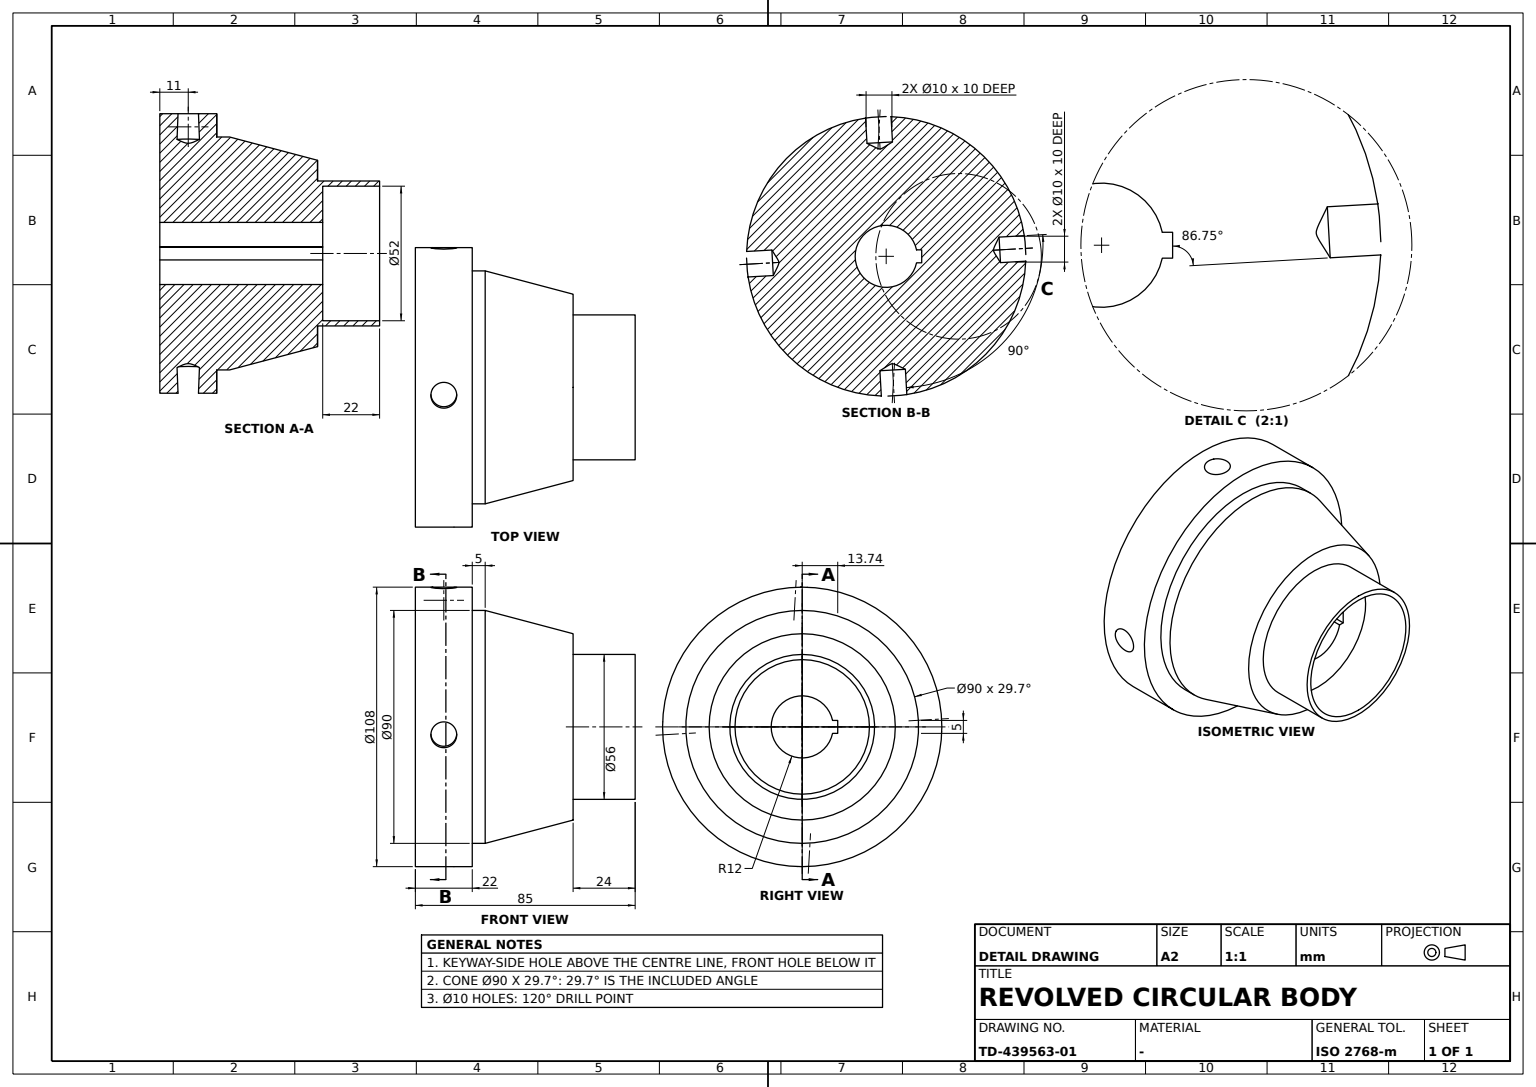
ISO-10303-21;
HEADER;
FILE_DESCRIPTION((''),'2;1');
FILE_NAME('','',(''),(''),'','','');
FILE_SCHEMA(('AUTOMOTIVE_DESIGN'));
ENDSEC;
DATA;
#1=APPLICATION_CONTEXT('');
#2=PRODUCT_CONTEXT('',#1,'mechanical');
#3=PRODUCT('','','',(#2));
#4=PRODUCT_DEFINITION_FORMATION('','',#3);
#5=PRODUCT_DEFINITION_CONTEXT('',#1,'design');
#6=PRODUCT_DEFINITION('','',#4,#5);
#7=PRODUCT_DEFINITION_SHAPE('','',#6);
#8=(LENGTH_UNIT()NAMED_UNIT(*)SI_UNIT(.MILLI.,.METRE.));
#9=(NAMED_UNIT(*)PLANE_ANGLE_UNIT()SI_UNIT($,.RADIAN.));
#10=(NAMED_UNIT(*)SI_UNIT($,.STERADIAN.)SOLID_ANGLE_UNIT());
#11=UNCERTAINTY_MEASURE_WITH_UNIT(LENGTH_MEASURE(0.005),#8,'distance_accuracy_value','');
#12=(GEOMETRIC_REPRESENTATION_CONTEXT(3)GLOBAL_UNCERTAINTY_ASSIGNED_CONTEXT((#11))GLOBAL_UNIT_ASSIGNED_CONTEXT((#8,#9,#10))REPRESENTATION_CONTEXT('',''));
#13=CARTESIAN_POINT('',(-78.387913,-0.666342,53.995889));
#14=VERTEX_POINT('',#13);
#15=CARTESIAN_POINT('',(-79.315768,-4.629244,53.854393));
#16=CARTESIAN_POINT('',(-78.86274,-0.407001,54.04207));
#17=CARTESIAN_POINT('',(-75.560747,2.259197,53.952659));
#18=CARTESIAN_POINT('',(-71.347706,1.80512,53.979216));
#19=CARTESIAN_POINT('',(-68.68427,-1.499404,54.032185));
#20=CARTESIAN_POINT('',(-69.13719,-5.715656,53.740509));
#21=CARTESIAN_POINT('',(-72.439195,-8.354711,53.349717));
#22=CARTESIAN_POINT('',(-76.652299,-7.906564,53.427525));
#23=B_SPLINE_CURVE_WITH_KNOTS('',3,(#15,#16,#17,#18,#19,#20,#21,#22,#15,#16,#17),.UNSPECIFIED.,.T.,.F.,(1,1,1,1,1,1,1,1,1,1,1,1,1,1,1),(-0.01172778,-0.00781852,-0.00390926,0.,0.00390926,0.00781852,0.01172778,0.01563704,0.0195463,0.02345556,0.02736482,0.03127408,0.035183339,0.039092599,0.043001859),.UNSPECIFIED.);
#24=EDGE_CURVE('',#14,#14,#23,.T.);
#25=ORIENTED_EDGE('',*,*,#24,.F.);
#26=EDGE_LOOP('',(#25));
#27=FACE_BOUND('',#26,.T.);
#28=CARTESIAN_POINT('',(-74.,-7.487428,43.6456));
#29=VERTEX_POINT('',#28);
#30=CARTESIAN_POINT('',(-74.,-2.495477,43.929177));
#31=DIRECTION('',(0.,-0.056715376,0.998390388));
#32=DIRECTION('',(0.,-0.998390388,-0.056715376));
#33=AXIS2_PLACEMENT_3D('',#30,#31,#32);
#34=CIRCLE('',#33,5.);
#35=EDGE_CURVE('',#29,#29,#34,.F.);
#36=ORIENTED_EDGE('',*,*,#35,.T.);
#37=EDGE_LOOP('',(#36));
#38=FACE_BOUND('',#37,.T.);
#39=CARTESIAN_POINT('',(-74.,-3.056959,53.813242));
#40=DIRECTION('',(0.,0.056715376,-0.998390388));
#41=DIRECTION('',(1.,0.,0.));
#42=AXIS2_PLACEMENT_3D('',#39,#40,#41);
#43=CYLINDRICAL_SURFACE('',#42,5.);
#44=ADVANCED_FACE('',(#27,#38),#43,.F.);
#45=ORIENTED_EDGE('',*,*,#35,.F.);
#46=EDGE_LOOP('',(#45));
#47=FACE_BOUND('',#46,.T.);
#48=CARTESIAN_POINT('',(-74.,-2.331753,41.047072));
#49=VERTEX_POINT('',#48);
#50=VERTEX_LOOP('',#49);
#51=FACE_BOUND('',#50,.T.);
#52=AXIS2_PLACEMENT_3D('',#48,#31,#41);
#53=CONICAL_SURFACE('',#52,0.,1.047197551);
#54=ADVANCED_FACE('',(#47,#51),#53,.F.);
#55=CARTESIAN_POINT('',(-74.,43.6456,7.487428));
#56=VERTEX_POINT('',#55);
#57=CARTESIAN_POINT('',(-74.,43.929177,2.495477));
#58=DIRECTION('',(0.,0.998390388,0.056715376));
#59=AXIS2_PLACEMENT_3D('',#57,#58,#31);
#60=CIRCLE('',#59,5.);
#61=EDGE_CURVE('',#56,#56,#60,.F.);
#62=ORIENTED_EDGE('',*,*,#61,.F.);
#63=EDGE_LOOP('',(#62));
#64=FACE_BOUND('',#63,.T.);
#65=CARTESIAN_POINT('',(-74.,41.047072,2.331753));
#66=VERTEX_POINT('',#65);
#67=VERTEX_LOOP('',#66);
#68=FACE_BOUND('',#67,.T.);
#69=AXIS2_PLACEMENT_3D('',#65,#58,#41);
#70=CONICAL_SURFACE('',#69,0.,1.047197551);
#71=ADVANCED_FACE('',(#64,#68),#70,.F.);
#72=CARTESIAN_POINT('',(-24.,0.,28.));
#73=VERTEX_POINT('',#72);
#74=CARTESIAN_POINT('',(-24.,0.,0.));
#75=DIRECTION('',(-1.,0.,0.));
#76=DIRECTION('',(0.,0.,1.));
#77=AXIS2_PLACEMENT_3D('',#74,#75,#76);
#78=CIRCLE('',#77,28.);
#79=EDGE_CURVE('',#73,#73,#78,.T.);
#80=ORIENTED_EDGE('',*,*,#79,.F.);
#81=EDGE_LOOP('',(#80));
#82=FACE_BOUND('',#81,.T.);
#83=CARTESIAN_POINT('',(0.,0.,28.));
#84=VERTEX_POINT('',#83);
#85=CARTESIAN_POINT('',(0.,0.,0.));
#86=AXIS2_PLACEMENT_3D('',#85,#75,#76);
#87=CIRCLE('',#86,28.);
#88=EDGE_CURVE('',#84,#84,#87,.T.);
#89=ORIENTED_EDGE('',*,*,#88,.T.);
#90=EDGE_LOOP('',(#89));
#91=FACE_BOUND('',#90,.T.);
#92=CARTESIAN_POINT('',(-42.5,0.,0.));
#93=DIRECTION('',(0.,1.,0.));
#94=AXIS2_PLACEMENT_3D('',#92,#75,#93);
#95=CYLINDRICAL_SURFACE('',#94,28.);
#96=ADVANCED_FACE('',(#82,#91),#95,.T.);
#97=CARTESIAN_POINT('',(-24.,0.,36.));
#98=VERTEX_POINT('',#97);
#99=CIRCLE('',#77,36.);
#100=EDGE_CURVE('',#98,#98,#99,.T.);
#101=ORIENTED_EDGE('',*,*,#100,.F.);
#102=EDGE_LOOP('',(#101));
#103=FACE_BOUND('',#102,.T.);
#104=ORIENTED_EDGE('',*,*,#79,.T.);
#105=EDGE_LOOP('',(#104));
#106=FACE_BOUND('',#105,.T.);
#107=AXIS2_PLACEMENT_3D('',#97,#75,#93);
#108=PLANE('',#107);
#109=ADVANCED_FACE('',(#103,#106),#108,.F.);
#110=ORIENTED_EDGE('',*,*,#100,.T.);
#111=EDGE_LOOP('',(#110));
#112=FACE_BOUND('',#111,.T.);
#113=CARTESIAN_POINT('',(-58.,0.,45.));
#114=VERTEX_POINT('',#113);
#115=CARTESIAN_POINT('',(-58.,0.,0.));
#116=AXIS2_PLACEMENT_3D('',#115,#75,#76);
#117=CIRCLE('',#116,45.);
#118=EDGE_CURVE('',#114,#114,#117,.T.);
#119=ORIENTED_EDGE('',*,*,#118,.F.);
#120=EDGE_LOOP('',(#119));
#121=FACE_BOUND('',#120,.T.);
#122=AXIS2_PLACEMENT_3D('',#74,#75,#93);
#123=CONICAL_SURFACE('',#122,36.,0.258770892);
#124=ADVANCED_FACE('',(#112,#121),#123,.T.);
#125=CARTESIAN_POINT('',(-74.,2.331753,-41.047072));
#126=VERTEX_POINT('',#125);
#127=VERTEX_LOOP('',#126);
#128=FACE_BOUND('',#127,.T.);
#129=CARTESIAN_POINT('',(-74.,7.487428,-43.6456));
#130=VERTEX_POINT('',#129);
#131=CARTESIAN_POINT('',(-74.,2.495477,-43.929177));
#132=AXIS2_PLACEMENT_3D('',#131,#40,#58);
#133=CIRCLE('',#132,5.);
#134=EDGE_CURVE('',#130,#130,#133,.F.);
#135=ORIENTED_EDGE('',*,*,#134,.F.);
#136=EDGE_LOOP('',(#135));
#137=FACE_BOUND('',#136,.T.);
#138=AXIS2_PLACEMENT_3D('',#125,#40,#41);
#139=CONICAL_SURFACE('',#138,0.,1.047197551);
#140=ADVANCED_FACE('',(#128,#137),#139,.F.);
#141=CARTESIAN_POINT('',(-78.387913,53.995889,0.666342));
#142=VERTEX_POINT('',#141);
#143=CARTESIAN_POINT('',(-79.315768,53.854393,4.629244));
#144=CARTESIAN_POINT('',(-78.86274,54.04207,0.407001));
#145=CARTESIAN_POINT('',(-75.560747,53.952659,-2.259197));
#146=CARTESIAN_POINT('',(-71.347706,53.979216,-1.80512));
#147=CARTESIAN_POINT('',(-68.68427,54.032185,1.499404));
#148=CARTESIAN_POINT('',(-69.13719,53.740509,5.715656));
#149=CARTESIAN_POINT('',(-72.439195,53.349717,8.354711));
#150=CARTESIAN_POINT('',(-76.652299,53.427525,7.906564));
#151=B_SPLINE_CURVE_WITH_KNOTS('',3,(#143,#144,#145,#146,#147,#148,#149,#150,#143,#144,#145),.UNSPECIFIED.,.T.,.F.,(1,1,1,1,1,1,1,1,1,1,1,1,1,1,1),(-0.01172778,-0.00781852,-0.00390926,0.,0.00390926,0.00781852,0.01172778,0.01563704,0.0195463,0.02345556,0.02736482,0.03127408,0.035183339,0.039092599,0.043001859),.UNSPECIFIED.);
#152=EDGE_CURVE('',#142,#142,#151,.T.);
#153=ORIENTED_EDGE('',*,*,#152,.F.);
#154=EDGE_LOOP('',(#153));
#155=FACE_BOUND('',#154,.T.);
#156=ORIENTED_EDGE('',*,*,#61,.T.);
#157=EDGE_LOOP('',(#156));
#158=FACE_BOUND('',#157,.T.);
#159=CARTESIAN_POINT('',(-74.,53.813242,3.056959));
#160=AXIS2_PLACEMENT_3D('',#159,#32,#41);
#161=CYLINDRICAL_SURFACE('',#160,5.);
#162=ADVANCED_FACE('',(#155,#158),#161,.F.);
#163=CARTESIAN_POINT('',(-78.387913,0.666342,-53.995889));
#164=VERTEX_POINT('',#163);
#165=CARTESIAN_POINT('',(-79.315768,4.629244,-53.854393));
#166=CARTESIAN_POINT('',(-78.86274,0.407001,-54.04207));
#167=CARTESIAN_POINT('',(-75.560747,-2.259197,-53.952659));
#168=CARTESIAN_POINT('',(-71.347706,-1.80512,-53.979216));
#169=CARTESIAN_POINT('',(-68.68427,1.499404,-54.032185));
#170=CARTESIAN_POINT('',(-69.13719,5.715656,-53.740509));
#171=CARTESIAN_POINT('',(-72.439195,8.354711,-53.349717));
#172=CARTESIAN_POINT('',(-76.652299,7.906564,-53.427525));
#173=B_SPLINE_CURVE_WITH_KNOTS('',3,(#165,#166,#167,#168,#169,#170,#171,#172,#165,#166,#167),.UNSPECIFIED.,.T.,.F.,(1,1,1,1,1,1,1,1,1,1,1,1,1,1,1),(-0.01172778,-0.00781852,-0.00390926,0.,0.00390926,0.00781852,0.01172778,0.01563704,0.0195463,0.02345556,0.02736482,0.03127408,0.035183339,0.039092599,0.043001859),.UNSPECIFIED.);
#174=EDGE_CURVE('',#164,#164,#173,.T.);
#175=ORIENTED_EDGE('',*,*,#174,.T.);
#176=EDGE_LOOP('',(#175));
#177=FACE_BOUND('',#176,.T.);
#178=CARTESIAN_POINT('',(-63.,0.,54.));
#179=VERTEX_POINT('',#178);
#180=CARTESIAN_POINT('',(-63.,0.,0.));
#181=AXIS2_PLACEMENT_3D('',#180,#75,#76);
#182=CIRCLE('',#181,54.);
#183=EDGE_CURVE('',#179,#179,#182,.T.);
#184=ORIENTED_EDGE('',*,*,#183,.T.);
#185=EDGE_LOOP('',(#184));
#186=FACE_BOUND('',#185,.T.);
#187=CARTESIAN_POINT('',(-85.,0.,54.));
#188=VERTEX_POINT('',#187);
#189=CARTESIAN_POINT('',(-85.,0.,0.));
#190=AXIS2_PLACEMENT_3D('',#189,#75,#76);
#191=CIRCLE('',#190,54.);
#192=EDGE_CURVE('',#188,#188,#191,.T.);
#193=ORIENTED_EDGE('',*,*,#192,.F.);
#194=EDGE_LOOP('',(#193));
#195=FACE_BOUND('',#194,.T.);
#196=ORIENTED_EDGE('',*,*,#152,.T.);
#197=EDGE_LOOP('',(#196));
#198=FACE_BOUND('',#197,.T.);
#199=CARTESIAN_POINT('',(-78.387913,-53.995889,-0.666342));
#200=VERTEX_POINT('',#199);
#201=CARTESIAN_POINT('',(-79.315768,-53.854393,-4.629244));
#202=CARTESIAN_POINT('',(-78.86274,-54.04207,-0.407001));
#203=CARTESIAN_POINT('',(-75.560747,-53.952659,2.259197));
#204=CARTESIAN_POINT('',(-71.347706,-53.979216,1.80512));
#205=CARTESIAN_POINT('',(-68.68427,-54.032185,-1.499404));
#206=CARTESIAN_POINT('',(-69.13719,-53.740509,-5.715656));
#207=CARTESIAN_POINT('',(-72.439195,-53.349717,-8.354711));
#208=CARTESIAN_POINT('',(-76.652299,-53.427525,-7.906564));
#209=B_SPLINE_CURVE_WITH_KNOTS('',3,(#201,#202,#203,#204,#205,#206,#207,#208,#201,#202,#203),.UNSPECIFIED.,.T.,.F.,(1,1,1,1,1,1,1,1,1,1,1,1,1,1,1),(-0.01172778,-0.00781852,-0.00390926,0.,0.00390926,0.00781852,0.01172778,0.01563704,0.0195463,0.02345556,0.02736482,0.03127408,0.035183339,0.039092599,0.043001859),.UNSPECIFIED.);
#210=EDGE_CURVE('',#200,#200,#209,.T.);
#211=ORIENTED_EDGE('',*,*,#210,.T.);
#212=EDGE_LOOP('',(#211));
#213=FACE_BOUND('',#212,.T.);
#214=ORIENTED_EDGE('',*,*,#24,.T.);
#215=EDGE_LOOP('',(#214));
#216=FACE_BOUND('',#215,.T.);
#217=CYLINDRICAL_SURFACE('',#94,54.);
#218=ADVANCED_FACE('',(#177,#186,#195,#198,#213,#216),#217,.T.);
#219=CARTESIAN_POINT('',(-74.,-43.6456,-7.487428));
#220=VERTEX_POINT('',#219);
#221=CARTESIAN_POINT('',(-74.,-43.929177,-2.495477));
#222=AXIS2_PLACEMENT_3D('',#221,#32,#40);
#223=CIRCLE('',#222,5.);
#224=EDGE_CURVE('',#220,#220,#223,.F.);
#225=ORIENTED_EDGE('',*,*,#224,.F.);
#226=EDGE_LOOP('',(#225));
#227=FACE_BOUND('',#226,.T.);
#228=CARTESIAN_POINT('',(-74.,-41.047072,-2.331753));
#229=VERTEX_POINT('',#228);
#230=VERTEX_LOOP('',#229);
#231=FACE_BOUND('',#230,.T.);
#232=AXIS2_PLACEMENT_3D('',#228,#32,#41);
#233=CONICAL_SURFACE('',#232,0.,1.047197551);
#234=ADVANCED_FACE('',(#227,#231),#233,.F.);
#235=ORIENTED_EDGE('',*,*,#192,.T.);
#236=EDGE_LOOP('',(#235));
#237=FACE_BOUND('',#236,.T.);
#238=CARTESIAN_POINT('',(-85.,11.736695,-2.5));
#239=VERTEX_POINT('',#238);
#240=CARTESIAN_POINT('',(-85.,11.736695,2.5));
#241=VERTEX_POINT('',#240);
#242=CIRCLE('',#190,12.);
#243=EDGE_CURVE('',#239,#241,#242,.T.);
#244=ORIENTED_EDGE('',*,*,#243,.F.);
#245=CARTESIAN_POINT('',(-85.,13.736695,-2.5));
#246=VERTEX_POINT('',#245);
#247=CARTESIAN_POINT('',(-85.,0.,-2.5));
#248=DIRECTION('',(0.,-1.,0.));
#249=VECTOR('',#248,1000.);
#250=LINE('',#247,#249);
#251=EDGE_CURVE('',#246,#239,#250,.T.);
#252=ORIENTED_EDGE('',*,*,#251,.F.);
#253=CARTESIAN_POINT('',(-85.,13.736695,2.5));
#254=VERTEX_POINT('',#253);
#255=CARTESIAN_POINT('',(-85.,13.736695,54.));
#256=DIRECTION('',(0.,0.,-1.));
#257=VECTOR('',#256,1000.);
#258=LINE('',#255,#257);
#259=EDGE_CURVE('',#254,#246,#258,.T.);
#260=ORIENTED_EDGE('',*,*,#259,.F.);
#261=CARTESIAN_POINT('',(-85.,0.,2.5));
#262=VECTOR('',#93,1000.);
#263=LINE('',#261,#262);
#264=EDGE_CURVE('',#241,#254,#263,.T.);
#265=ORIENTED_EDGE('',*,*,#264,.F.);
#266=EDGE_LOOP('',(#244,#252,#260,#265));
#267=FACE_BOUND('',#266,.T.);
#268=AXIS2_PLACEMENT_3D('',#187,#75,#93);
#269=PLANE('',#268);
#270=ADVANCED_FACE('',(#237,#267),#269,.T.);
#271=CARTESIAN_POINT('',(-22.,13.736695,2.5));
#272=VERTEX_POINT('',#271);
#273=VECTOR('',#75,1000.);
#274=LINE('',#271,#273);
#275=EDGE_CURVE('',#272,#254,#274,.T.);
#276=ORIENTED_EDGE('',*,*,#275,.F.);
#277=CARTESIAN_POINT('',(-22.,11.736695,2.5));
#278=VERTEX_POINT('',#277);
#279=LINE('',#277,#262);
#280=EDGE_CURVE('',#278,#272,#279,.T.);
#281=ORIENTED_EDGE('',*,*,#280,.F.);
#282=VECTOR('',#41,1000.);
#283=LINE('',#277,#282);
#284=EDGE_CURVE('',#278,#241,#283,.F.);
#285=ORIENTED_EDGE('',*,*,#284,.T.);
#286=ORIENTED_EDGE('',*,*,#264,.T.);
#287=EDGE_LOOP('',(#276,#281,#285,#286));
#288=FACE_BOUND('',#287,.T.);
#289=AXIS2_PLACEMENT_3D('',#277,#76,#93);
#290=PLANE('',#289);
#291=ADVANCED_FACE('',(#288),#290,.F.);
#292=CARTESIAN_POINT('',(-22.,13.736695,-2.5));
#293=VERTEX_POINT('',#292);
#294=CARTESIAN_POINT('',(-22.,11.736695,-2.5));
#295=VERTEX_POINT('',#294);
#296=LINE('',#292,#249);
#297=EDGE_CURVE('',#293,#295,#296,.T.);
#298=ORIENTED_EDGE('',*,*,#297,.T.);
#299=CARTESIAN_POINT('',(-22.,0.,0.));
#300=AXIS2_PLACEMENT_3D('',#299,#41,#256);
#301=CIRCLE('',#300,12.);
#302=EDGE_CURVE('',#278,#295,#301,.T.);
#303=ORIENTED_EDGE('',*,*,#302,.F.);
#304=ORIENTED_EDGE('',*,*,#280,.T.);
#305=LINE('',#271,#257);
#306=EDGE_CURVE('',#272,#293,#305,.T.);
#307=ORIENTED_EDGE('',*,*,#306,.T.);
#308=EDGE_LOOP('',(#298,#303,#304,#307));
#309=FACE_BOUND('',#308,.T.);
#310=CARTESIAN_POINT('',(-22.,0.,-26.));
#311=VERTEX_POINT('',#310);
#312=CIRCLE('',#300,26.);
#313=EDGE_CURVE('',#311,#311,#312,.T.);
#314=ORIENTED_EDGE('',*,*,#313,.T.);
#315=EDGE_LOOP('',(#314));
#316=FACE_BOUND('',#315,.T.);
#317=AXIS2_PLACEMENT_3D('',#299,#41,#93);
#318=PLANE('',#317);
#319=ADVANCED_FACE('',(#309,#316),#318,.T.);
#320=CARTESIAN_POINT('',(-63.,0.,45.));
#321=VERTEX_POINT('',#320);
#322=CIRCLE('',#181,45.);
#323=EDGE_CURVE('',#321,#321,#322,.T.);
#324=ORIENTED_EDGE('',*,*,#323,.F.);
#325=EDGE_LOOP('',(#324));
#326=FACE_BOUND('',#325,.T.);
#327=ORIENTED_EDGE('',*,*,#118,.T.);
#328=EDGE_LOOP('',(#327));
#329=FACE_BOUND('',#328,.T.);
#330=CYLINDRICAL_SURFACE('',#94,45.);
#331=ADVANCED_FACE('',(#326,#329),#330,.T.);
#332=ORIENTED_EDGE('',*,*,#224,.T.);
#333=EDGE_LOOP('',(#332));
#334=FACE_BOUND('',#333,.T.);
#335=ORIENTED_EDGE('',*,*,#210,.F.);
#336=EDGE_LOOP('',(#335));
#337=FACE_BOUND('',#336,.T.);
#338=ADVANCED_FACE('',(#334,#337),#161,.F.);
#339=CARTESIAN_POINT('',(0.,0.,26.));
#340=VERTEX_POINT('',#339);
#341=CIRCLE('',#86,26.);
#342=EDGE_CURVE('',#340,#340,#341,.F.);
#343=ORIENTED_EDGE('',*,*,#342,.F.);
#344=EDGE_LOOP('',(#343));
#345=FACE_BOUND('',#344,.T.);
#346=ORIENTED_EDGE('',*,*,#88,.F.);
#347=EDGE_LOOP('',(#346));
#348=FACE_BOUND('',#347,.T.);
#349=AXIS2_PLACEMENT_3D('',#85,#75,#93);
#350=PLANE('',#349);
#351=ADVANCED_FACE('',(#345,#348),#350,.F.);
#352=ORIENTED_EDGE('',*,*,#284,.F.);
#353=ORIENTED_EDGE('',*,*,#302,.T.);
#354=LINE('',#294,#282);
#355=EDGE_CURVE('',#295,#239,#354,.F.);
#356=ORIENTED_EDGE('',*,*,#355,.T.);
#357=ORIENTED_EDGE('',*,*,#243,.T.);
#358=EDGE_LOOP('',(#352,#353,#356,#357));
#359=FACE_BOUND('',#358,.T.);
#360=CARTESIAN_POINT('',(-54.16,0.,0.));
#361=AXIS2_PLACEMENT_3D('',#360,#41,#93);
#362=CYLINDRICAL_SURFACE('',#361,12.);
#363=ADVANCED_FACE('',(#359),#362,.F.);
#364=ORIENTED_EDGE('',*,*,#183,.F.);
#365=EDGE_LOOP('',(#364));
#366=FACE_BOUND('',#365,.T.);
#367=ORIENTED_EDGE('',*,*,#323,.T.);
#368=EDGE_LOOP('',(#367));
#369=FACE_BOUND('',#368,.T.);
#370=AXIS2_PLACEMENT_3D('',#320,#75,#93);
#371=PLANE('',#370);
#372=ADVANCED_FACE('',(#366,#369),#371,.F.);
#373=ORIENTED_EDGE('',*,*,#174,.F.);
#374=EDGE_LOOP('',(#373));
#375=FACE_BOUND('',#374,.T.);
#376=ORIENTED_EDGE('',*,*,#134,.T.);
#377=EDGE_LOOP('',(#376));
#378=FACE_BOUND('',#377,.T.);
#379=ADVANCED_FACE('',(#375,#378),#43,.F.);
#380=ORIENTED_EDGE('',*,*,#297,.F.);
#381=LINE('',#292,#273);
#382=EDGE_CURVE('',#293,#246,#381,.T.);
#383=ORIENTED_EDGE('',*,*,#382,.T.);
#384=ORIENTED_EDGE('',*,*,#251,.T.);
#385=ORIENTED_EDGE('',*,*,#355,.F.);
#386=EDGE_LOOP('',(#380,#383,#384,#385));
#387=FACE_BOUND('',#386,.T.);
#388=AXIS2_PLACEMENT_3D('',#292,#256,#248);
#389=PLANE('',#388);
#390=ADVANCED_FACE('',(#387),#389,.F.);
#391=ORIENTED_EDGE('',*,*,#382,.F.);
#392=ORIENTED_EDGE('',*,*,#306,.F.);
#393=ORIENTED_EDGE('',*,*,#275,.T.);
#394=ORIENTED_EDGE('',*,*,#259,.T.);
#395=EDGE_LOOP('',(#391,#392,#393,#394));
#396=FACE_BOUND('',#395,.T.);
#397=AXIS2_PLACEMENT_3D('',#271,#93,#256);
#398=PLANE('',#397);
#399=ADVANCED_FACE('',(#396),#398,.F.);
#400=ORIENTED_EDGE('',*,*,#313,.F.);
#401=EDGE_LOOP('',(#400));
#402=FACE_BOUND('',#401,.T.);
#403=ORIENTED_EDGE('',*,*,#342,.T.);
#404=EDGE_LOOP('',(#403));
#405=FACE_BOUND('',#404,.T.);
#406=CARTESIAN_POINT('',(-11.,0.,0.));
#407=AXIS2_PLACEMENT_3D('',#406,#41,#93);
#408=CYLINDRICAL_SURFACE('',#407,26.);
#409=ADVANCED_FACE('',(#402,#405),#408,.F.);
#410=CLOSED_SHELL('',(#44,#54,#71,#96,#109,#124,#140,#162,#218,#234,#270,#291,#319,#331,#338,#351,#363,#372,#379,#390,#399,#409));
#411=MANIFOLD_SOLID_BREP('',#410);
#412=ADVANCED_BREP_SHAPE_REPRESENTATION('',(#411),#12);
#413=SHAPE_DEFINITION_REPRESENTATION(#7,#412);
ENDSEC;
END-ISO-10303-21;
